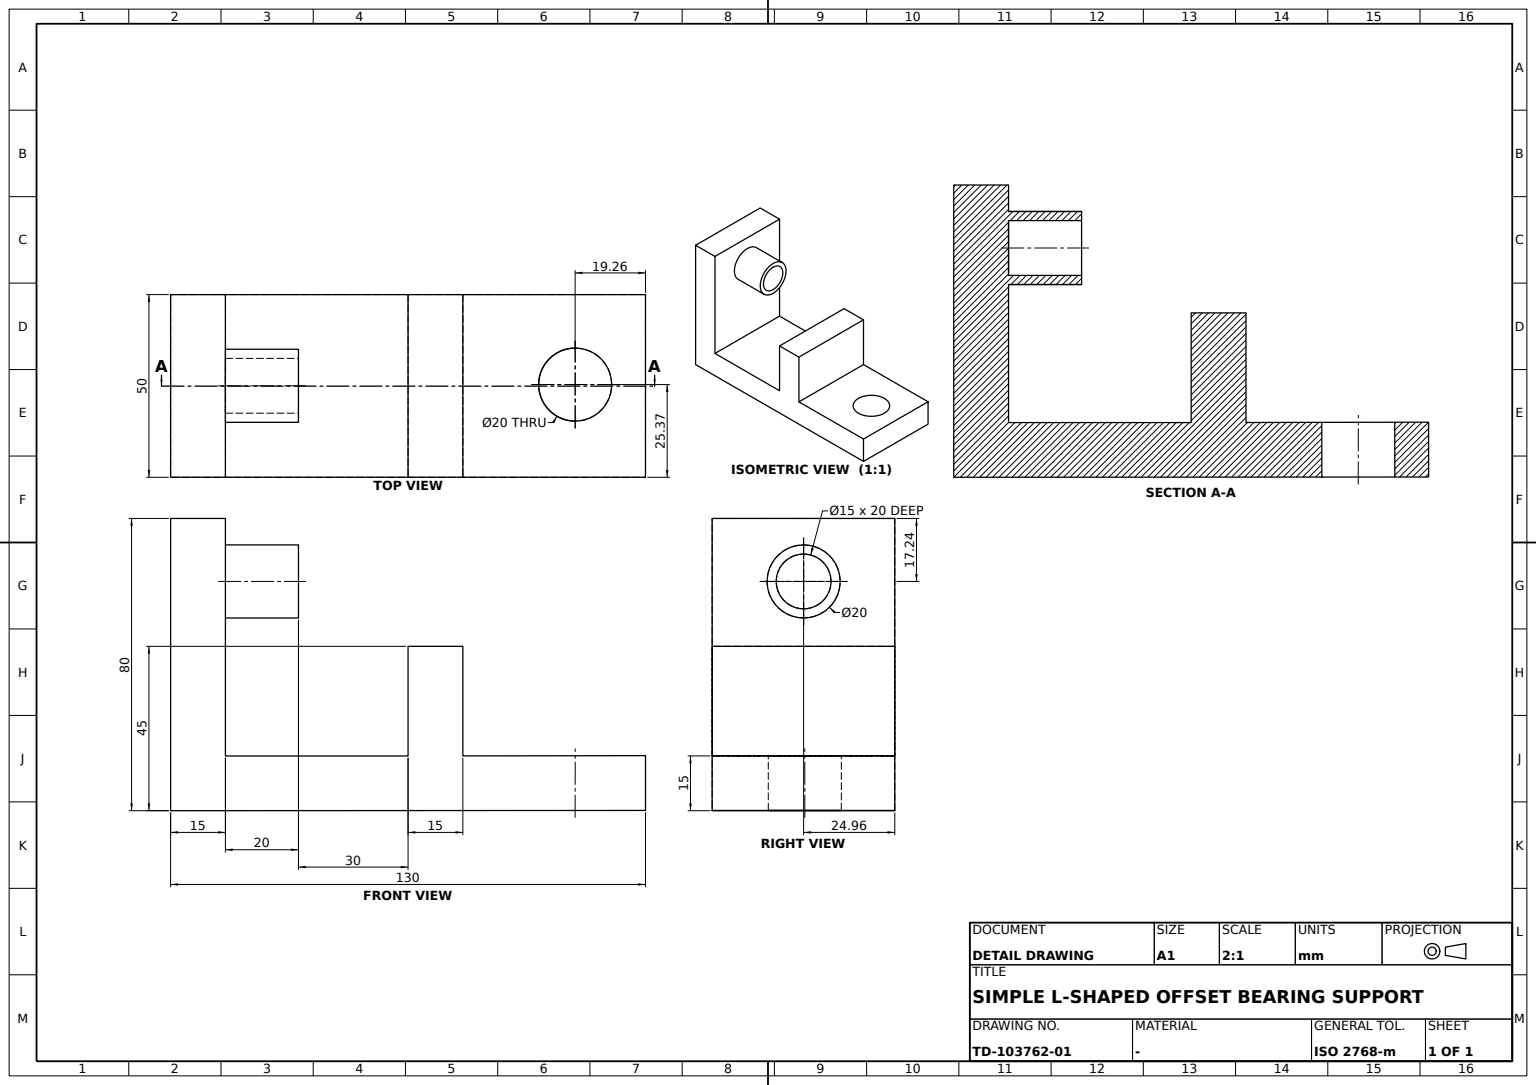
ISO-10303-21;
HEADER;
FILE_DESCRIPTION((''),'2;1');
FILE_NAME('','',(''),(''),'','','');
FILE_SCHEMA(('AUTOMOTIVE_DESIGN'));
ENDSEC;
DATA;
#1=APPLICATION_CONTEXT('');
#2=PRODUCT_CONTEXT('',#1,'mechanical');
#3=PRODUCT('','','',(#2));
#4=PRODUCT_DEFINITION_FORMATION('','',#3);
#5=PRODUCT_DEFINITION_CONTEXT('',#1,'design');
#6=PRODUCT_DEFINITION('','',#4,#5);
#7=PRODUCT_DEFINITION_SHAPE('','',#6);
#8=(LENGTH_UNIT()NAMED_UNIT(*)SI_UNIT(.MILLI.,.METRE.));
#9=(NAMED_UNIT(*)PLANE_ANGLE_UNIT()SI_UNIT($,.RADIAN.));
#10=(NAMED_UNIT(*)SI_UNIT($,.STERADIAN.)SOLID_ANGLE_UNIT());
#11=UNCERTAINTY_MEASURE_WITH_UNIT(LENGTH_MEASURE(0.005),#8,'distance_accuracy_value','');
#12=(GEOMETRIC_REPRESENTATION_CONTEXT(3)GLOBAL_UNCERTAINTY_ASSIGNED_CONTEXT((#11))GLOBAL_UNIT_ASSIGNED_CONTEXT((#8,#9,#10))REPRESENTATION_CONTEXT('',''));
#13=CARTESIAN_POINT('',(24.632402,100.760595,0.056765));
#14=VERTEX_POINT('',#13);
#15=CARTESIAN_POINT('',(24.632402,110.760598,0.062399));
#16=DIRECTION('',(0.,0.000563365,-0.999999841));
#17=DIRECTION('',(0.,-0.999999841,-0.000563365));
#18=AXIS2_PLACEMENT_3D('',#15,#16,#17);
#19=ELLIPSE('',#18,10.000004,10.);
#20=EDGE_CURVE('',#14,#14,#19,.F.);
#21=ORIENTED_EDGE('',*,*,#20,.F.);
#22=EDGE_LOOP('',(#21));
#23=FACE_BOUND('',#22,.T.);
#24=CARTESIAN_POINT('',(24.632402,100.737995,15.029068));
#25=VERTEX_POINT('',#24);
#26=CARTESIAN_POINT('',(24.632402,110.737984,15.044163));
#27=DIRECTION('',(0.,-0.00150944,0.999998861));
#28=DIRECTION('',(0.,-0.999998861,-0.00150944));
#29=AXIS2_PLACEMENT_3D('',#26,#27,#28);
#30=CIRCLE('',#29,10.);
#31=EDGE_CURVE('',#25,#25,#30,.T.);
#32=ORIENTED_EDGE('',*,*,#31,.T.);
#33=EDGE_LOOP('',(#32));
#34=FACE_BOUND('',#33,.T.);
#35=CARTESIAN_POINT('',(24.632402,110.753078,5.044174));
#36=DIRECTION('',(1.,0.,0.));
#37=AXIS2_PLACEMENT_3D('',#35,#27,#36);
#38=CYLINDRICAL_SURFACE('',#37,10.);
#39=ADVANCED_FACE('',(#23,#34),#38,.F.);
#40=CARTESIAN_POINT('',(50.,80.000036,14.997765));
#41=VERTEX_POINT('',#40);
#42=CARTESIAN_POINT('',(50.,80.000036,44.997765));
#43=VERTEX_POINT('',#42);
#44=CARTESIAN_POINT('',(50.,80.000036,0.));
#45=DIRECTION('',(0.,0.,1.));
#46=VECTOR('',#45,1000.);
#47=LINE('',#44,#46);
#48=EDGE_CURVE('',#41,#43,#47,.T.);
#49=ORIENTED_EDGE('',*,*,#48,.F.);
#50=CARTESIAN_POINT('',(0.,80.000036,14.997765));
#51=VERTEX_POINT('',#50);
#52=VECTOR('',#36,1000.);
#53=LINE('',#50,#52);
#54=EDGE_CURVE('',#51,#41,#53,.T.);
#55=ORIENTED_EDGE('',*,*,#54,.F.);
#56=CARTESIAN_POINT('',(0.,80.000036,44.997765));
#57=VERTEX_POINT('',#56);
#58=CARTESIAN_POINT('',(0.,80.000036,0.));
#59=LINE('',#58,#46);
#60=EDGE_CURVE('',#51,#57,#59,.T.);
#61=ORIENTED_EDGE('',*,*,#60,.T.);
#62=LINE('',#56,#52);
#63=EDGE_CURVE('',#57,#43,#62,.T.);
#64=ORIENTED_EDGE('',*,*,#63,.T.);
#65=EDGE_LOOP('',(#49,#55,#61,#64));
#66=FACE_BOUND('',#65,.T.);
#67=DIRECTION('',(0.,1.,0.));
#68=AXIS2_PLACEMENT_3D('',#50,#67,#45);
#69=PLANE('',#68);
#70=ADVANCED_FACE('',(#66),#69,.T.);
#71=CARTESIAN_POINT('',(24.959404,15.,55.256771));
#72=VERTEX_POINT('',#71);
#73=CARTESIAN_POINT('',(24.959404,15.,62.756771));
#74=DIRECTION('',(0.,-1.,0.));
#75=DIRECTION('',(0.,0.,-1.));
#76=AXIS2_PLACEMENT_3D('',#73,#74,#75);
#77=CIRCLE('',#76,7.5);
#78=EDGE_CURVE('',#72,#72,#77,.F.);
#79=ORIENTED_EDGE('',*,*,#78,.T.);
#80=EDGE_LOOP('',(#79));
#81=FACE_BOUND('',#80,.T.);
#82=CARTESIAN_POINT('',(0.,15.,80.));
#83=AXIS2_PLACEMENT_3D('',#82,#74,#75);
#84=PLANE('',#83);
#85=ADVANCED_FACE('',(#81),#84,.F.);
#86=ORIENTED_EDGE('',*,*,#20,.T.);
#87=EDGE_LOOP('',(#86));
#88=FACE_BOUND('',#87,.T.);
#89=CARTESIAN_POINT('',(0.,129.999979,0.073237));
#90=VERTEX_POINT('',#89);
#91=CARTESIAN_POINT('',(50.,129.999979,0.073237));
#92=VERTEX_POINT('',#91);
#93=LINE('',#89,#52);
#94=EDGE_CURVE('',#90,#92,#93,.T.);
#95=ORIENTED_EDGE('',*,*,#94,.T.);
#96=CARTESIAN_POINT('',(50.,0.,0.));
#97=VERTEX_POINT('',#96);
#98=DIRECTION('',(0.,0.999999841,0.000563365));
#99=VECTOR('',#98,1000.);
#100=LINE('',#96,#99);
#101=EDGE_CURVE('',#97,#92,#100,.T.);
#102=ORIENTED_EDGE('',*,*,#101,.F.);
#103=CARTESIAN_POINT('',(0.,0.,0.));
#104=VERTEX_POINT('',#103);
#105=LINE('',#103,#52);
#106=EDGE_CURVE('',#104,#97,#105,.T.);
#107=ORIENTED_EDGE('',*,*,#106,.F.);
#108=LINE('',#103,#99);
#109=EDGE_CURVE('',#104,#90,#108,.T.);
#110=ORIENTED_EDGE('',*,*,#109,.T.);
#111=EDGE_LOOP('',(#95,#102,#107,#110));
#112=FACE_BOUND('',#111,.T.);
#113=AXIS2_PLACEMENT_3D('',#103,#16,#98);
#114=PLANE('',#113);
#115=ADVANCED_FACE('',(#88,#112),#114,.T.);
#116=CARTESIAN_POINT('',(0.,129.999979,15.073237));
#117=VERTEX_POINT('',#116);
#118=CARTESIAN_POINT('',(50.,129.999979,15.073237));
#119=VERTEX_POINT('',#118);
#120=LINE('',#116,#52);
#121=EDGE_CURVE('',#117,#119,#120,.T.);
#122=ORIENTED_EDGE('',*,*,#121,.T.);
#123=CARTESIAN_POINT('',(50.,129.999979,0.));
#124=LINE('',#123,#46);
#125=EDGE_CURVE('',#92,#119,#124,.T.);
#126=ORIENTED_EDGE('',*,*,#125,.F.);
#127=ORIENTED_EDGE('',*,*,#94,.F.);
#128=CARTESIAN_POINT('',(0.,129.999979,0.));
#129=LINE('',#128,#46);
#130=EDGE_CURVE('',#90,#117,#129,.T.);
#131=ORIENTED_EDGE('',*,*,#130,.T.);
#132=EDGE_LOOP('',(#122,#126,#127,#131));
#133=FACE_BOUND('',#132,.T.);
#134=AXIS2_PLACEMENT_3D('',#89,#67,#45);
#135=PLANE('',#134);
#136=ADVANCED_FACE('',(#133),#135,.T.);
#137=CARTESIAN_POINT('',(50.,65.000036,14.975124));
#138=VERTEX_POINT('',#137);
#139=CARTESIAN_POINT('',(50.,15.,14.975124));
#140=VERTEX_POINT('',#139);
#141=CARTESIAN_POINT('',(50.,0.,14.975124));
#142=VECTOR('',#74,1000.);
#143=LINE('',#141,#142);
#144=EDGE_CURVE('',#138,#140,#143,.T.);
#145=ORIENTED_EDGE('',*,*,#144,.F.);
#146=CARTESIAN_POINT('',(0.,65.000036,14.975124));
#147=VERTEX_POINT('',#146);
#148=LINE('',#146,#52);
#149=EDGE_CURVE('',#147,#138,#148,.T.);
#150=ORIENTED_EDGE('',*,*,#149,.F.);
#151=CARTESIAN_POINT('',(0.,15.,14.975124));
#152=VERTEX_POINT('',#151);
#153=CARTESIAN_POINT('',(0.,0.,14.975124));
#154=LINE('',#153,#142);
#155=EDGE_CURVE('',#147,#152,#154,.T.);
#156=ORIENTED_EDGE('',*,*,#155,.T.);
#157=LINE('',#151,#52);
#158=EDGE_CURVE('',#152,#140,#157,.T.);
#159=ORIENTED_EDGE('',*,*,#158,.T.);
#160=EDGE_LOOP('',(#145,#150,#156,#159));
#161=FACE_BOUND('',#160,.T.);
#162=AXIS2_PLACEMENT_3D('',#146,#45,#74);
#163=PLANE('',#162);
#164=ADVANCED_FACE('',(#161),#163,.T.);
#165=CARTESIAN_POINT('',(0.,-0.022456,14.876976));
#166=VECTOR('',#28,1000.);
#167=LINE('',#165,#166);
#168=EDGE_CURVE('',#117,#51,#167,.T.);
#169=ORIENTED_EDGE('',*,*,#168,.F.);
#170=ORIENTED_EDGE('',*,*,#130,.F.);
#171=ORIENTED_EDGE('',*,*,#109,.F.);
#172=CARTESIAN_POINT('',(0.,0.,80.));
#173=VERTEX_POINT('',#172);
#174=LINE('',#103,#46);
#175=EDGE_CURVE('',#104,#173,#174,.T.);
#176=ORIENTED_EDGE('',*,*,#175,.T.);
#177=VERTEX_POINT('',#82);
#178=VECTOR('',#67,1000.);
#179=LINE('',#172,#178);
#180=EDGE_CURVE('',#173,#177,#179,.T.);
#181=ORIENTED_EDGE('',*,*,#180,.T.);
#182=CARTESIAN_POINT('',(0.,15.,0.));
#183=VECTOR('',#75,1000.);
#184=LINE('',#182,#183);
#185=EDGE_CURVE('',#177,#152,#184,.T.);
#186=ORIENTED_EDGE('',*,*,#185,.T.);
#187=ORIENTED_EDGE('',*,*,#155,.F.);
#188=CARTESIAN_POINT('',(0.,65.000036,44.997765));
#189=VERTEX_POINT('',#188);
#190=CARTESIAN_POINT('',(0.,65.000036,0.));
#191=LINE('',#190,#183);
#192=EDGE_CURVE('',#189,#147,#191,.T.);
#193=ORIENTED_EDGE('',*,*,#192,.F.);
#194=CARTESIAN_POINT('',(0.,0.,44.997765));
#195=LINE('',#194,#142);
#196=EDGE_CURVE('',#57,#189,#195,.T.);
#197=ORIENTED_EDGE('',*,*,#196,.F.);
#198=ORIENTED_EDGE('',*,*,#60,.F.);
#199=EDGE_LOOP('',(#169,#170,#171,#176,#181,#186,#187,#193,#197,#198));
#200=FACE_BOUND('',#199,.T.);
#201=AXIS2_PLACEMENT_3D('',#103,#36,#67);
#202=PLANE('',#201);
#203=ADVANCED_FACE('',(#200),#202,.F.);
#204=ORIENTED_EDGE('',*,*,#106,.T.);
#205=CARTESIAN_POINT('',(50.,0.,80.));
#206=VERTEX_POINT('',#205);
#207=LINE('',#96,#46);
#208=EDGE_CURVE('',#97,#206,#207,.T.);
#209=ORIENTED_EDGE('',*,*,#208,.T.);
#210=LINE('',#172,#52);
#211=EDGE_CURVE('',#173,#206,#210,.T.);
#212=ORIENTED_EDGE('',*,*,#211,.F.);
#213=ORIENTED_EDGE('',*,*,#175,.F.);
#214=EDGE_LOOP('',(#204,#209,#212,#213));
#215=FACE_BOUND('',#214,.T.);
#216=AXIS2_PLACEMENT_3D('',#103,#67,#45);
#217=PLANE('',#216);
#218=ADVANCED_FACE('',(#215),#217,.F.);
#219=ORIENTED_EDGE('',*,*,#208,.F.);
#220=ORIENTED_EDGE('',*,*,#101,.T.);
#221=ORIENTED_EDGE('',*,*,#125,.T.);
#222=CARTESIAN_POINT('',(50.,-0.022456,14.876976));
#223=LINE('',#222,#166);
#224=EDGE_CURVE('',#119,#41,#223,.T.);
#225=ORIENTED_EDGE('',*,*,#224,.T.);
#226=ORIENTED_EDGE('',*,*,#48,.T.);
#227=CARTESIAN_POINT('',(50.,65.000036,44.997765));
#228=VERTEX_POINT('',#227);
#229=CARTESIAN_POINT('',(50.,0.,44.997765));
#230=LINE('',#229,#142);
#231=EDGE_CURVE('',#43,#228,#230,.T.);
#232=ORIENTED_EDGE('',*,*,#231,.T.);
#233=CARTESIAN_POINT('',(50.,65.000036,0.));
#234=LINE('',#233,#183);
#235=EDGE_CURVE('',#228,#138,#234,.T.);
#236=ORIENTED_EDGE('',*,*,#235,.T.);
#237=ORIENTED_EDGE('',*,*,#144,.T.);
#238=CARTESIAN_POINT('',(50.,15.,80.));
#239=VERTEX_POINT('',#238);
#240=CARTESIAN_POINT('',(50.,15.,0.));
#241=LINE('',#240,#183);
#242=EDGE_CURVE('',#239,#140,#241,.T.);
#243=ORIENTED_EDGE('',*,*,#242,.F.);
#244=LINE('',#205,#178);
#245=EDGE_CURVE('',#206,#239,#244,.T.);
#246=ORIENTED_EDGE('',*,*,#245,.F.);
#247=EDGE_LOOP('',(#219,#220,#221,#225,#226,#232,#236,#237,#243,#246));
#248=FACE_BOUND('',#247,.T.);
#249=AXIS2_PLACEMENT_3D('',#96,#36,#67);
#250=PLANE('',#249);
#251=ADVANCED_FACE('',(#248),#250,.T.);
#252=ORIENTED_EDGE('',*,*,#149,.T.);
#253=ORIENTED_EDGE('',*,*,#235,.F.);
#254=LINE('',#188,#52);
#255=EDGE_CURVE('',#189,#228,#254,.T.);
#256=ORIENTED_EDGE('',*,*,#255,.F.);
#257=ORIENTED_EDGE('',*,*,#192,.T.);
#258=EDGE_LOOP('',(#252,#253,#256,#257));
#259=FACE_BOUND('',#258,.T.);
#260=AXIS2_PLACEMENT_3D('',#188,#74,#75);
#261=PLANE('',#260);
#262=ADVANCED_FACE('',(#259),#261,.T.);
#263=ORIENTED_EDGE('',*,*,#196,.T.);
#264=ORIENTED_EDGE('',*,*,#255,.T.);
#265=ORIENTED_EDGE('',*,*,#231,.F.);
#266=ORIENTED_EDGE('',*,*,#63,.F.);
#267=EDGE_LOOP('',(#263,#264,#265,#266));
#268=FACE_BOUND('',#267,.T.);
#269=AXIS2_PLACEMENT_3D('',#56,#45,#74);
#270=PLANE('',#269);
#271=ADVANCED_FACE('',(#268),#270,.T.);
#272=CARTESIAN_POINT('',(24.959404,35.,72.756771));
#273=VERTEX_POINT('',#272);
#274=CARTESIAN_POINT('',(24.959404,35.,62.756771));
#275=AXIS2_PLACEMENT_3D('',#274,#67,#45);
#276=CIRCLE('',#275,10.);
#277=EDGE_CURVE('',#273,#273,#276,.T.);
#278=ORIENTED_EDGE('',*,*,#277,.T.);
#279=EDGE_LOOP('',(#278));
#280=FACE_BOUND('',#279,.T.);
#281=CARTESIAN_POINT('',(24.959404,35.,70.256771));
#282=VERTEX_POINT('',#281);
#283=CIRCLE('',#275,7.5);
#284=EDGE_CURVE('',#282,#282,#283,.T.);
#285=ORIENTED_EDGE('',*,*,#284,.F.);
#286=EDGE_LOOP('',(#285));
#287=FACE_BOUND('',#286,.T.);
#288=CARTESIAN_POINT('',(0.,35.,0.));
#289=DIRECTION('',(-1.,0.,0.));
#290=AXIS2_PLACEMENT_3D('',#288,#67,#289);
#291=PLANE('',#290);
#292=ADVANCED_FACE('',(#280,#287),#291,.T.);
#293=ORIENTED_EDGE('',*,*,#211,.T.);
#294=ORIENTED_EDGE('',*,*,#245,.T.);
#295=LINE('',#82,#52);
#296=EDGE_CURVE('',#177,#239,#295,.T.);
#297=ORIENTED_EDGE('',*,*,#296,.F.);
#298=ORIENTED_EDGE('',*,*,#180,.F.);
#299=EDGE_LOOP('',(#293,#294,#297,#298));
#300=FACE_BOUND('',#299,.T.);
#301=AXIS2_PLACEMENT_3D('',#172,#75,#67);
#302=PLANE('',#301);
#303=ADVANCED_FACE('',(#300),#302,.F.);
#304=ORIENTED_EDGE('',*,*,#158,.F.);
#305=ORIENTED_EDGE('',*,*,#185,.F.);
#306=ORIENTED_EDGE('',*,*,#296,.T.);
#307=ORIENTED_EDGE('',*,*,#242,.T.);
#308=EDGE_LOOP('',(#304,#305,#306,#307));
#309=FACE_BOUND('',#308,.T.);
#310=CARTESIAN_POINT('',(24.959404,15.,52.756771));
#311=VERTEX_POINT('',#310);
#312=CIRCLE('',#76,10.);
#313=EDGE_CURVE('',#311,#311,#312,.F.);
#314=ORIENTED_EDGE('',*,*,#313,.F.);
#315=EDGE_LOOP('',(#314));
#316=FACE_BOUND('',#315,.T.);
#317=ADVANCED_FACE('',(#309,#316),#84,.F.);
#318=ORIENTED_EDGE('',*,*,#277,.F.);
#319=EDGE_LOOP('',(#318));
#320=FACE_BOUND('',#319,.T.);
#321=ORIENTED_EDGE('',*,*,#313,.T.);
#322=EDGE_LOOP('',(#321));
#323=FACE_BOUND('',#322,.T.);
#324=CARTESIAN_POINT('',(24.959404,25.,62.756771));
#325=AXIS2_PLACEMENT_3D('',#324,#67,#289);
#326=CYLINDRICAL_SURFACE('',#325,10.);
#327=ADVANCED_FACE('',(#320,#323),#326,.T.);
#328=ORIENTED_EDGE('',*,*,#78,.F.);
#329=EDGE_LOOP('',(#328));
#330=FACE_BOUND('',#329,.T.);
#331=ORIENTED_EDGE('',*,*,#284,.T.);
#332=EDGE_LOOP('',(#331));
#333=FACE_BOUND('',#332,.T.);
#334=CYLINDRICAL_SURFACE('',#325,7.5);
#335=ADVANCED_FACE('',(#330,#333),#334,.F.);
#336=ORIENTED_EDGE('',*,*,#168,.T.);
#337=ORIENTED_EDGE('',*,*,#54,.T.);
#338=ORIENTED_EDGE('',*,*,#224,.F.);
#339=ORIENTED_EDGE('',*,*,#121,.F.);
#340=EDGE_LOOP('',(#336,#337,#338,#339));
#341=FACE_BOUND('',#340,.T.);
#342=ORIENTED_EDGE('',*,*,#31,.F.);
#343=EDGE_LOOP('',(#342));
#344=FACE_BOUND('',#343,.T.);
#345=AXIS2_PLACEMENT_3D('',#116,#27,#28);
#346=PLANE('',#345);
#347=ADVANCED_FACE('',(#341,#344),#346,.T.);
#348=CLOSED_SHELL('',(#39,#70,#85,#115,#136,#164,#203,#218,#251,#262,#271,#292,#303,#317,#327,#335,#347));
#349=MANIFOLD_SOLID_BREP('',#348);
#350=ADVANCED_BREP_SHAPE_REPRESENTATION('',(#349),#12);
#351=SHAPE_DEFINITION_REPRESENTATION(#7,#350);
ENDSEC;
END-ISO-10303-21;
